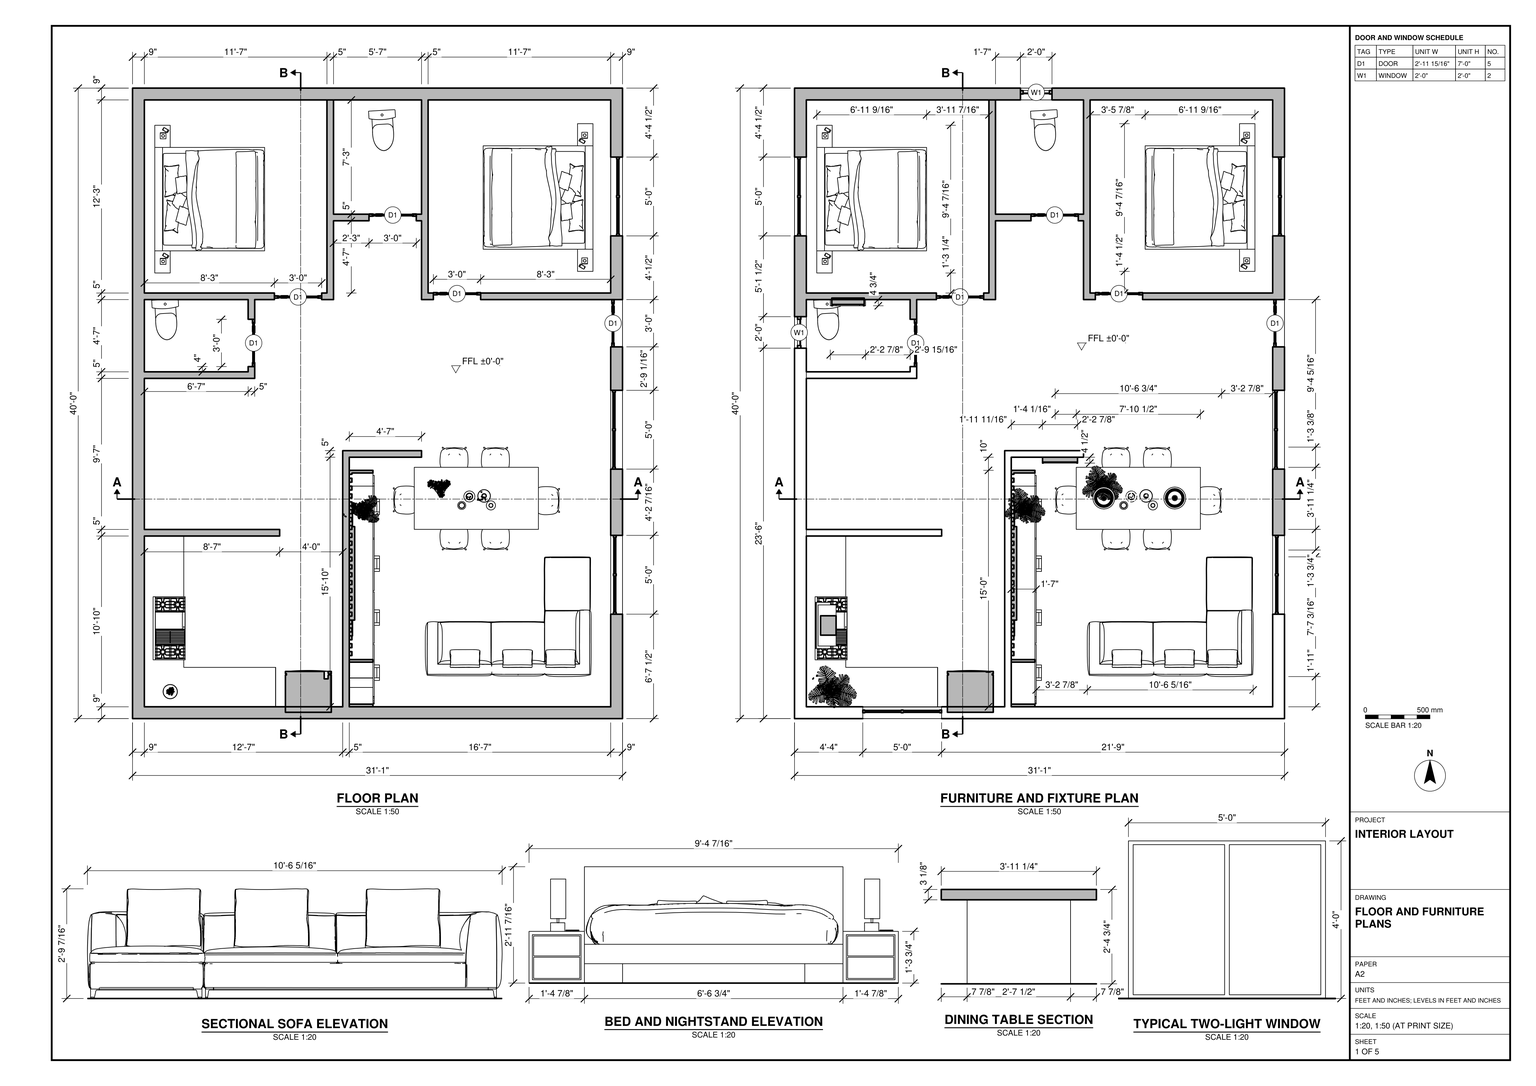
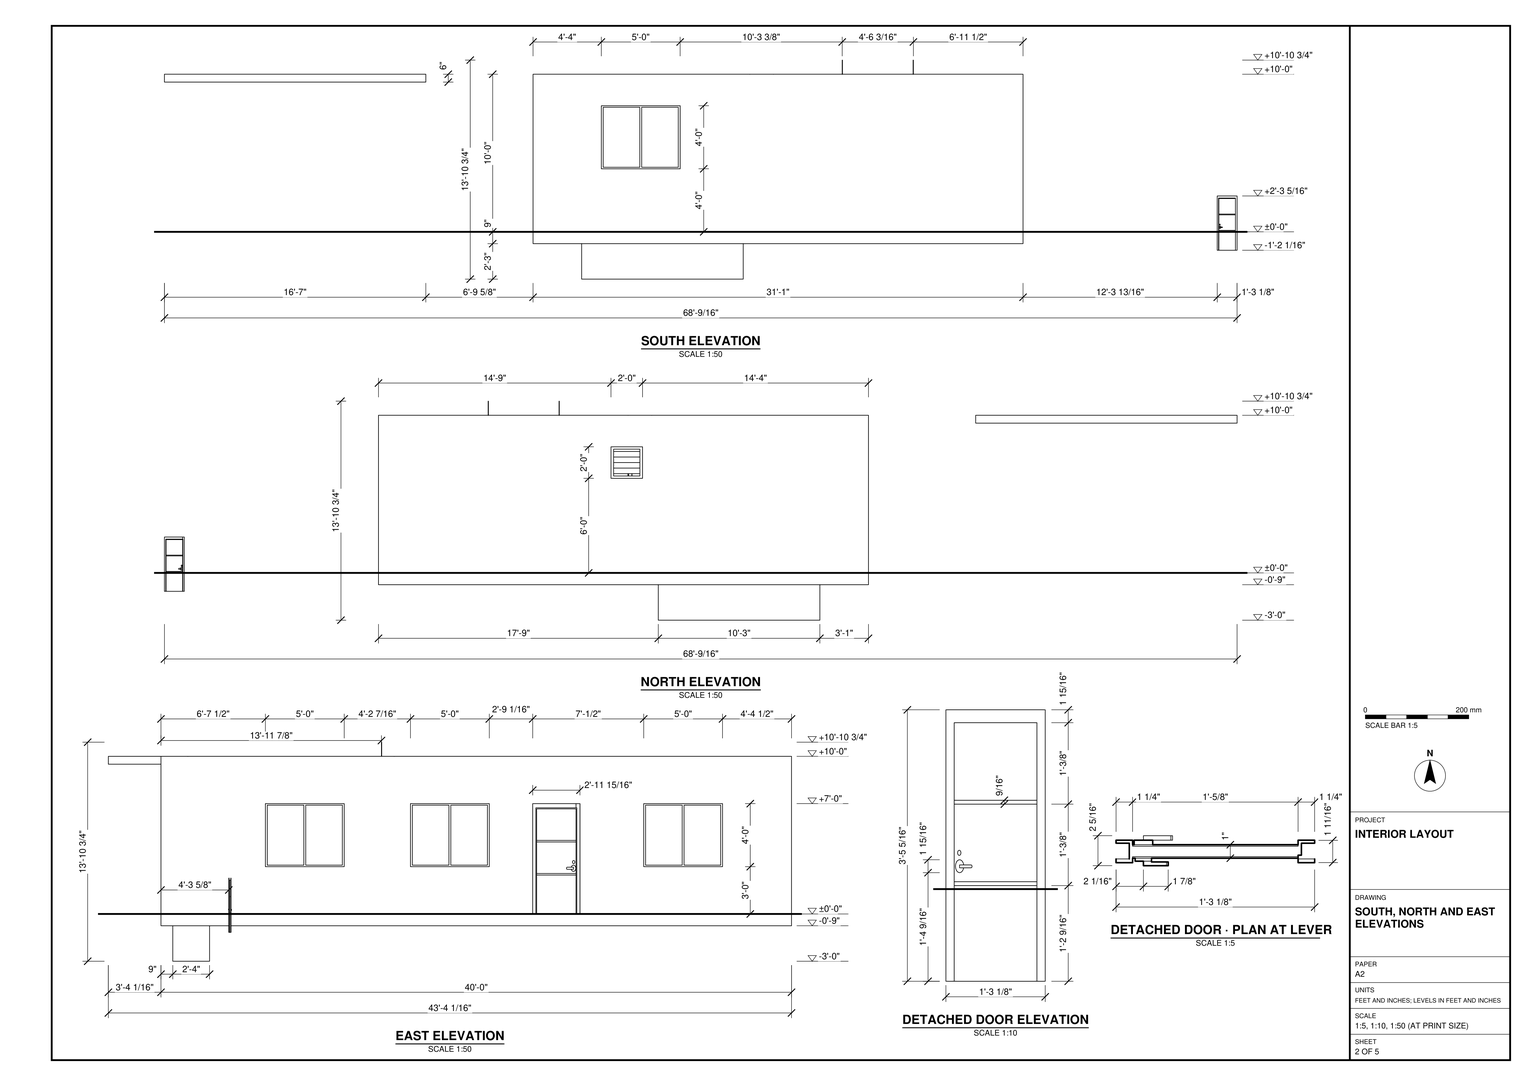
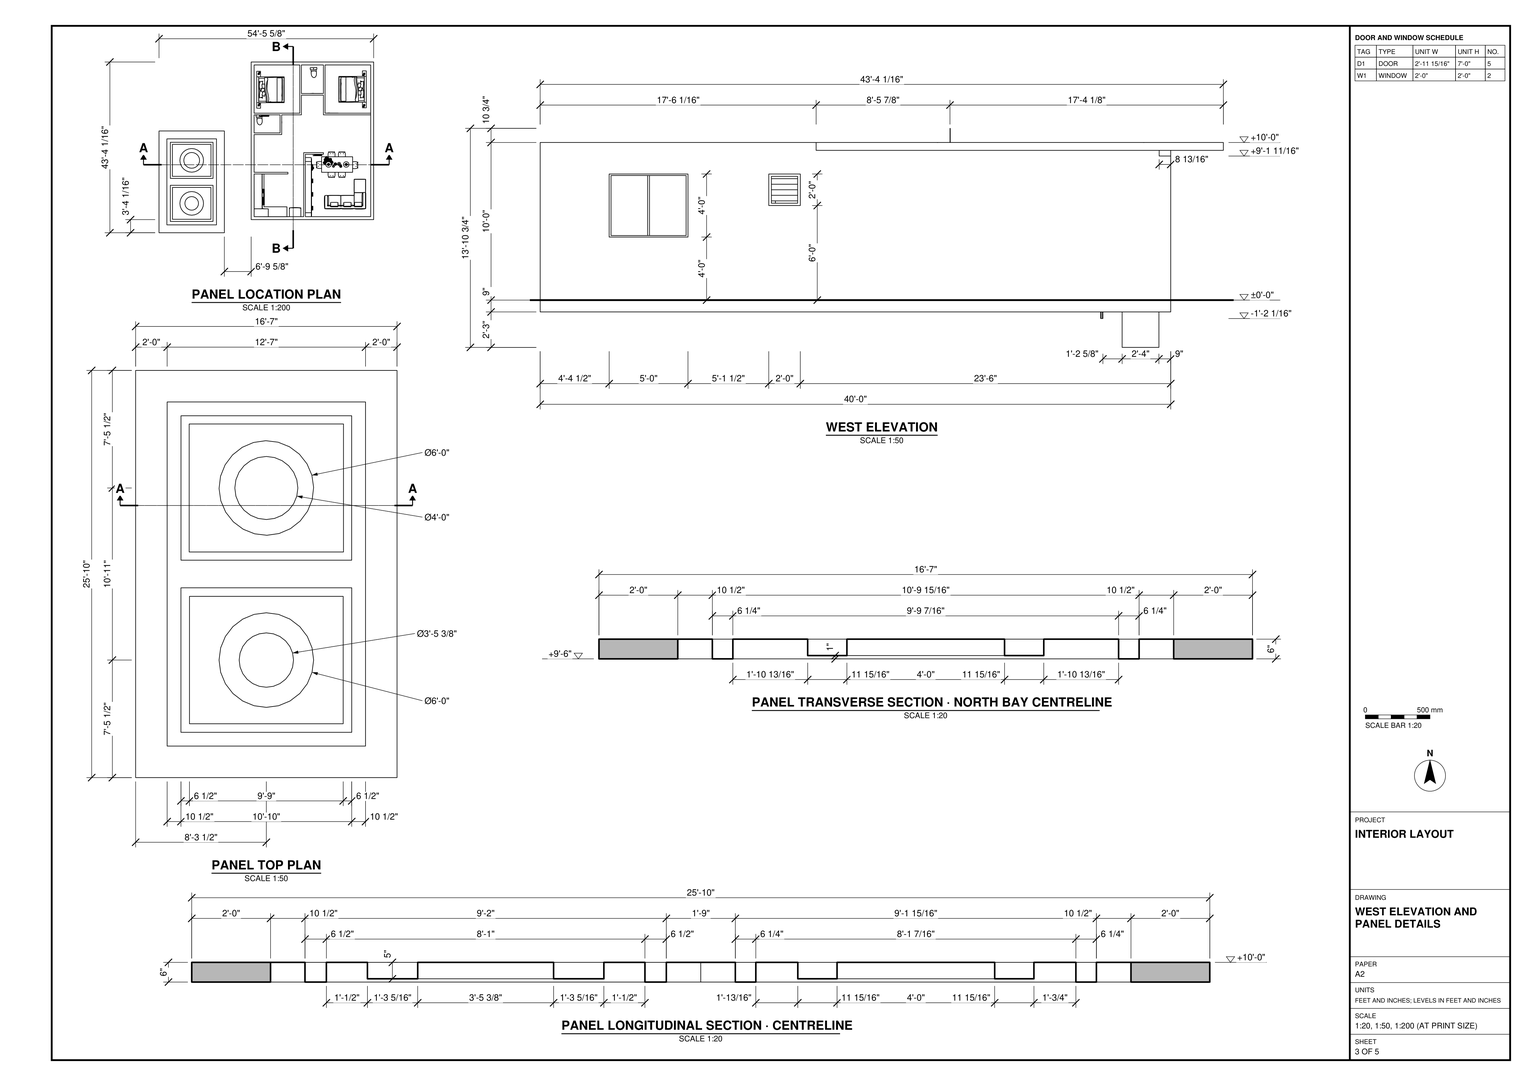
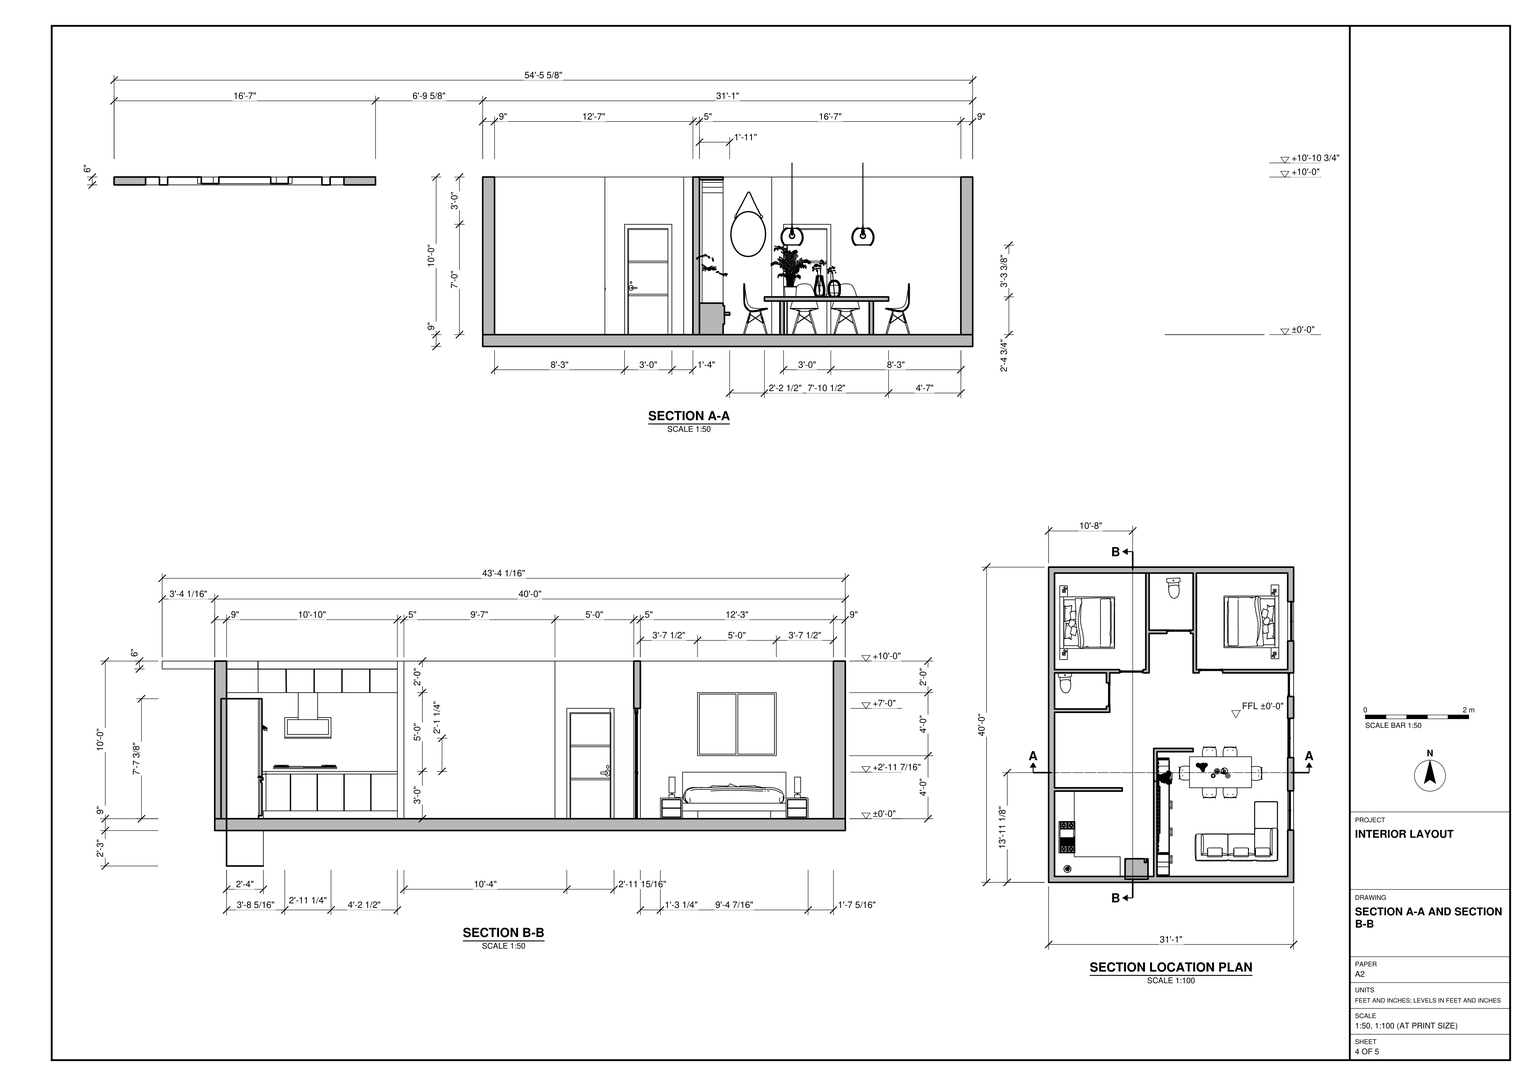
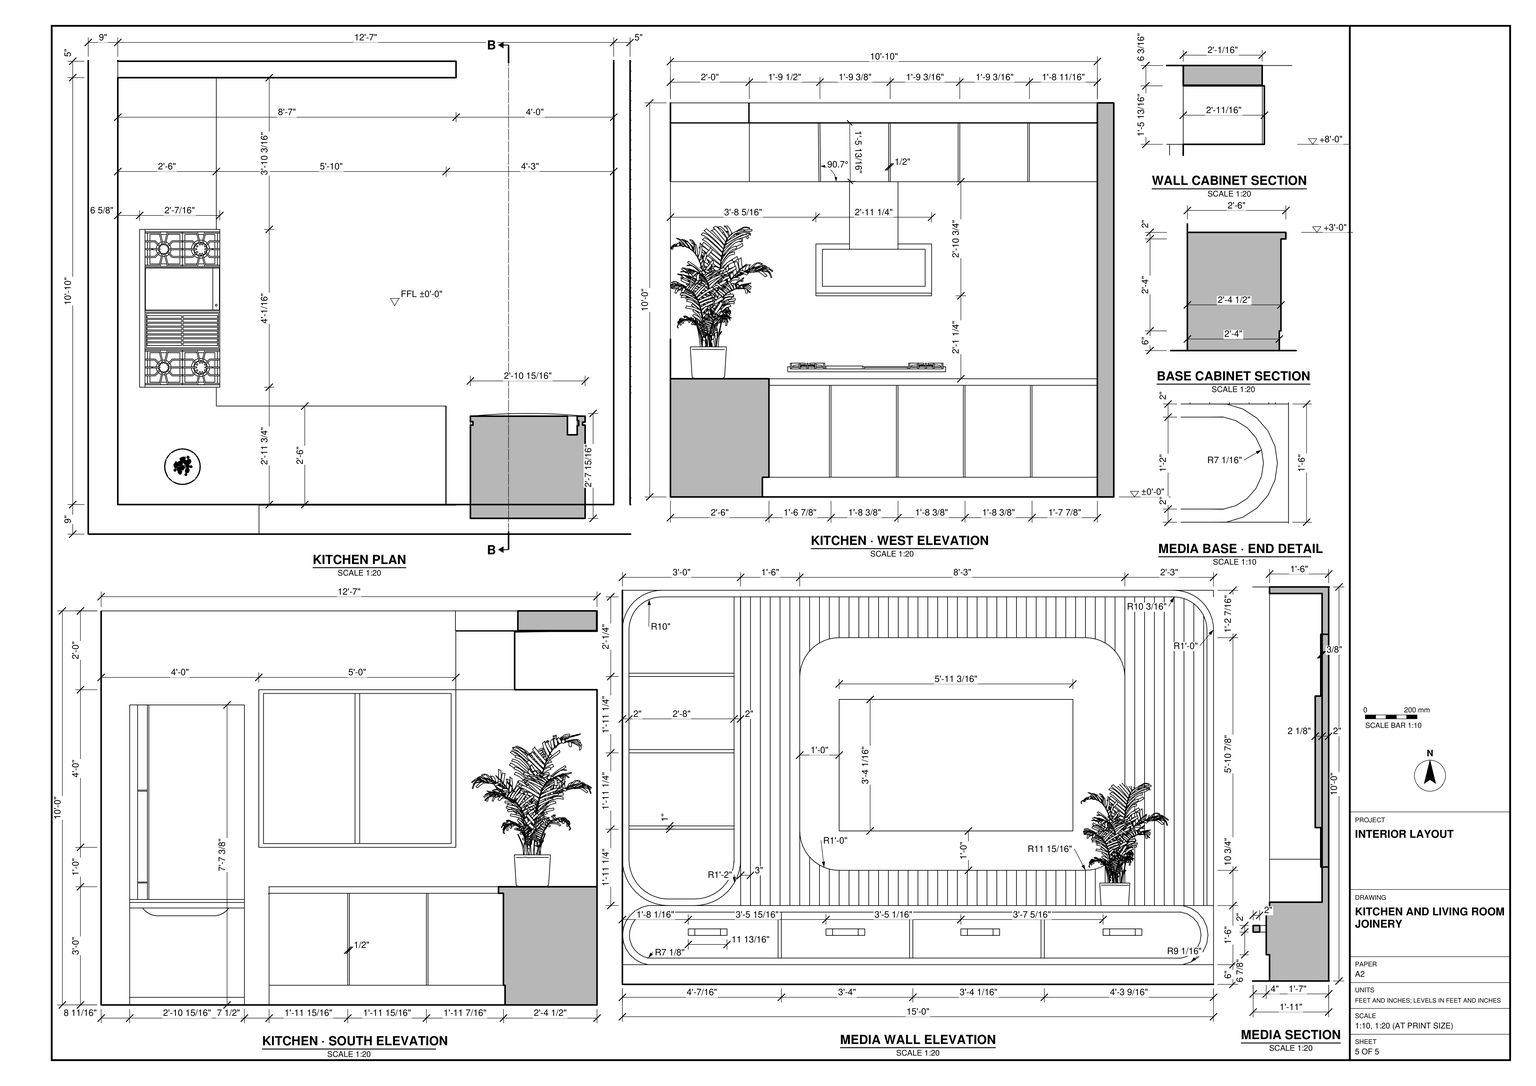
Build the interior in SketchUp from task_files/diagram_01.pdf. Work in feet and inches. Use the single finished floor level of ±0'-0". The shell measures 31'-1" east to west by 40'-0" north to south. Including the detached panel and door in their drawn positions, the overall model measures 68'-9/16" along X, 43'-4 1/16" along Y and 13'-10 3/4" along Z.

Model the floor slab, the 9" perimeter walls and the 5" partitions. Place the bedrooms in the north corners, with one toilet room between them and the other against the west wall. Follow the plans and elevations for the doors, the small high windows and the larger two-light windows. Fit out both bedrooms with beds and paired nightstands. In the southwest kitchen, arrange the counters, storage, sink and cooktop as drawn. Across the partition, place the living-area joinery, sectional sofa and dining table with chairs, keeping the passages clear as shown in plan.

Use the panel plan and sections to form the detached ceiling panel with its stepped rectangular bays and circular details. Set it west of the shell at the elevation shown, and place the separate small door east of the shell rather than fitting it into a wall. Decor and loose items, including plants, lamps, cushions and appliances, may be any suitable library components. Keep the shell elements and each furniture or joinery piece in separate groups or components, and use components for repeated parts. Save one SketchUp model as output_files/two_bedroom_interior_with_detached_ceiling_panel.skp.

# SketchUp Ruby script. Lengths in inches.
U = 1.inch
M = Sketchup.active_model
def pt(a) = Geom::Point3d.new(a.map { |v| v * U })
def face(e, loops, mat)
  f = e.add_face(loops[0].map { |a| pt(a) })
  loops[1..].each { |l| e.add_face(l.map { |a| pt(a) }).erase! }
  f.material = f.back_material = mat if mat
  f
end
# faces: each face lists its corners as indices into pts; further lists are holes
def faces(e, pts, list, mat = nil) = list.each { |f| face(e, (f[0].is_a?(Array) ? f : [f]).map { |l| l.map { |i| pts[i] } }, mat) }
# xy, xz, yz: faces in a plane at the given z, y or x. An outline is a flat list of corners, or four numbers for a rectangle; further outlines are holes
def ring(l) = l.size == 4 ? [[l[0], l[1]], [l[2], l[1]], [l[2], l[3]], [l[0], l[3]]] : l.each_slice(2).to_a
def flat(e, list, mat, &to3) = list.each { |f| face(e, (f[0].is_a?(Array) ? f : [f]).map { |l| ring(l).map { |u, v| to3.(u, v) } }, mat) }
def xy(e, z, list, mat = nil) = flat(e, list, mat) { |x, y| [x, y, z] }
def xz(e, y, list, mat = nil) = flat(e, list, mat) { |x, z| [x, y, z] }
def yz(e, x, list, mat = nil) = flat(e, list, mat) { |y, z| [x, y, z] }
def lines(e, pts, list) = list.each { |a, b| e.add_line(pt(pts[a]), pt(pts[b])) }
# prism: a flat outline (further loops are holes) pulled along v
def prism(e, loops, v, mat = nil)
  f = face(e, loops, mat); d = Geom::Vector3d.new(v.map { |x| x * U })
  f.pushpull(f.normal.samedirection?(d) ? d.length : -d.length)
end
def box(e, o, s, mat = nil) = prism(e, [[o, [o[0] + s[0], o[1], o[2]], [o[0] + s[0], o[1] + s[1], o[2]], [o[0], o[1] + s[1], o[2]]]], [0, 0, s[2]], mat)
def at(x, y, z, deg = 0) = Geom::Transformation.translation(pt([x, y, z])) * Geom::Transformation.rotation(ORIGIN, Z_AXIS, deg.degrees)
def axes(o, x, y, z) = Geom::Transformation.new([*x, 0, *y, 0, *z, 0, *pt(o).to_a, 1])
def part(name) = M.definitions.add(name)
# library, detail: a bought-in or finely detailed component or shape, given as its bounding box
def library(name, o, s) = part(name).tap { |d| box(d.entities, o, s) }
def detail(e, o, s) = box(e.add_group.entities, o, s)
def put(e, d, t, mat = nil) = e.add_instance(d, t).tap { |i| i.material = mat if mat }
def group(e, t, mat = nil) = e.add_group.tap { |g| g.transformation = t; g.material = mat if mat }.entities
root = M.entities
M.materials.add("[0008_LavenderBlush]").color = [255, 240, 245]
M.materials.add("[0022_Maroon]").color = [128, 0, 0]
M.materials.add("[0028_AntiqueWhite]").color = [250, 235, 215]
M.materials.add("[Carrera Marble]").color = [207, 207, 207]
M.materials.add("[Carrera Marble]1").color = [207, 207, 207]
M.materials.add("[Color_008]").color = [30, 30, 30]
M.materials.add("[Color_009]").color = [0, 0, 0]
M.materials.add("[Stone Marble]").color = [143, 138, 136]
M.materials.add("[Translucent Glass Gray]").color = [128, 128, 128]
M.materials["[Translucent Glass Gray]"].alpha = 0.5
M.materials.add("[Translucent Glass Tinted]1").color = [7, 201, 240]
M.materials["[Translucent Glass Tinted]1"].alpha = 0.48
M.materials.add("[Translucent_Glass_Gray]").color = [128, 128, 128]
M.materials["[Translucent_Glass_Gray]"].alpha = 0.5
M.materials.add("[Wood Cherry Original]").color = [152, 86, 42]
M.materials.add("[Wood Floor Parquet]").color = [145, 89, 39]
M.materials.add("[Wood Floor]").color = [155, 105, 61]
c1 = library("main+door",[0,-0.79,0],[47.24,7.88,82.68])
c2 = part("ventilator")
g1 = group(c2.entities,at(0,0,0))
xy(g1,0,[[0,0,24,1],[0,1,24,6.83]],"[Wood Floor Parquet]")
xy(g1,1.75,[[2,0,22,6.83]],"[Wood Floor Parquet]")
xy(g1,21.87,[[2,0,22,6.83]],"[Wood Cherry Original]")
xy(g1,23.62,[[0,0,24,1],[0,1,24,6.83]],"[Wood Floor Parquet]")
xz(g1,0,[[[0,0,24,23.62],[2,1.75,22,21.87]]],"[Wood Floor Parquet]")
xz(g1,6.83,[[[0,0,24,23.62],[2,1.75,22,21.87]]],"[Wood Cherry Original]")
yz(g1,0,[[0,0,1,23.62],[1,0,6.83,23.62]],"[Wood Floor Parquet]")
yz(g1,2,[[0,1.75,6.83,1.75,6.83,7.66,0,3.5],[0,3.5,6.83,7.66,6.83,11.8125,0,7.66],[0,7.66,6.83,11.8125,6.83,15.97,0,11.8125],[0,11.8125,6.83,15.97,6.83,20.12,0,15.97],[0,15.97,6.83,20.12,6.83,21.87,0,21.87]],"[Wood Floor Parquet]")
yz(g1,22,[[0,1.75,0,3.5,6.83,7.66,6.83,1.75],[0,3.5,0,7.66,6.83,11.8125,6.83,7.66],[0,7.66,0,11.8125,6.83,15.97,6.83,11.8125],[0,11.8125,0,15.97,6.83,20.12,6.83,15.97],[0,15.97,0,21.87,6.83,21.87,6.83,20.12]],"[Wood Floor Parquet]")
yz(g1,24,[[0,0,1,23.62],[1,0,6.83,23.62]],"[Wood Floor Parquet]")
p = [[2,0,3.5],[2,6.83,7.66],[22,6.83,7.66],[22,0,3.5],[2,6.83,11.8125],[2,0,7.66],
  [22,0,7.66],[22,6.83,11.8125],[2,0,11.8125],[2,6.83,15.97],[22,6.83,15.97],[22,0,11.8125],
  [2,6.83,20.12],[2,0,15.97],[22,0,15.97],[22,6.83,20.12]]
faces(g1,p,[[0,1,2,3],[4,5,6,7],[8,9,10,11]],"[Translucent Glass Tinted]1")
faces(g1,p,[[12,13,14,15]],"[Translucent Glass Gray]")
c3 = library("Double bed",[0,0,0],[83.59,112.46,35.43])
c4 = library("Gas cooktop",[0,0,34.52],[24.41,48.07,2.63])
c5 = part("Inclined chimney")
g2 = group(c5.entities,at(1.97,2.08,2.89))
xy(g2,0,[[0,7.9,31.3,13.68]])
xy(g2,11.29,[[0,0,31.3,13.68]])
xz(g2,13.68,[[0,0,31.3,11.29]])
yz(g2,0,[[7.9,0,0,11.29,13.68,11.29,13.68,0]])
yz(g2,31.3,[[7.9,0,13.68,0,13.68,11.29,0,11.29]])
g3 = group(c5.entities,at(0,9.85,0.4))
g4 = group(g3,at(0,0.61,0.43))
prism(g4,[[[35.24,0,0],[35.24,-3.39,4.84],[35.24,-3.58,4.7],[35.24,-0.29,0]]],[-35.24,0,0])
g5 = group(g3,at(0,-3.21,4.99))
prism(g5,[[[35.24,-0.2,-0.12],[35.24,-3.16,5],[0,-3.16,5],[0,-0.2,-0.12]]],[0,0.2,0.12])
g6 = group(g3,at(0,-6.27,10.27))
prism(g6,[[[35.24,-0.19,-0.14],[35.24,-3.58,4.7],[0,-3.58,4.7],[0,-0.19,-0.14]]],[0,0.19,0.14])
g7 = group(g3,at(0,0.61,0.43))
prism(g7,[[[35.24,0,0],[35.24,0.96,0],[35.24,-9.52,14.96],[35.24,-10.16,14.51]]],[-35.24,0,0])
g8 = group(c5.entities,at(10.24,3.95,20.8))
box(g8,[0,0,-6.62],[14.76,11.8125,20.56])
g9 = group(c5.entities,at(0,10.1,0))
prism(g9,[[[35.24,0.46,0],[35.24,1.33,0],[35.24,1.33,0.83],[35.24,1.01,0.83],[35.24,0.37,0.83],[35.24,0,0.83],[35.24,0,0.64]]],[-35.24,0,0])
c6 = part("Inclined+chimney")
put(c6.entities,c5,at(34.17,38.97,0.69))
c7 = library("Component\#33",[0,0,0],[60.64,55.48,158.625])
c8 = library("SKT_Nearly Natural 5' Kentia Palm Silk Tree",[-23.18,-17.61,0],[47.48,43.95,59.125])
c9 = library("CS300DRT",[0,0,0],[27.18,17.85,30.31])
c10 = library("Hanging wall mirror",[0,0,0],[26.88,1.18,49.49])
c11 = library("michel-club1 (1)",[-34.67,-0.85,-0.13],[126.28,91.17,33.41])
c12 = library("Modern+dining",[-0.9,-1.38,-0.1],[126.72,78.33,130.86])
c13 = library("Group\#13",[0,0,0],[23,180,120])
c14 = part("Group\#2")
xy(c14.entities,0,[[0,0,82.68,1.18]],"[Color_009]")
xy(c14.entities,1.97,[[1.97,0.98,40.35,1.18],[42.32,0.98,80.71,1.18]])
xy(c14.entities,1.97,[[1.97,0,40.35,0.3],[42.32,0,80.71,0.3]],"[Color_009]")
xy(c14.entities,80.71,[[1.97,0,40.35,0.3],[42.32,0,80.71,0.3],[1.97,0.3,40.35,0.98],[42.32,0.3,80.71,0.98],[1.97,0.98,40.35,1.18],
  [42.32,0.98,80.71,1.18]])
xy(c14.entities,82.68,[[0,0,82.68,1.18]],"[Color_008]")
xz(c14.entities,0,[[[0,0,82.68,82.68],[1.97,1.97,40.35,80.71],[42.32,1.97,80.71,80.71]]],"[Color_009]")
xz(c14.entities,0.3,[[1.97,1.97,40.35,80.71],[42.32,1.97,80.71,80.71]],"[Translucent_Glass_Gray]")
xz(c14.entities,0.98,[[1.97,1.97,40.35,80.71],[42.32,1.97,80.71,80.71]],"[Translucent_Glass_Gray]")
xz(c14.entities,1.18,[[[0,0,82.68,82.68],[1.97,1.97,80.71,80.71]],[40.35,1.97,42.32,80.71]],"[Color_009]")
yz(c14.entities,0,[[0,0,1.18,82.68]],"[Color_009]")
yz(c14.entities,1.97,[[0.98,1.97,1.18,80.71]])
yz(c14.entities,1.97,[[0,1.97,0.3,80.71]],"[Color_009]")
yz(c14.entities,40.35,[[0,1.97,0.3,80.71],[0.98,1.97,1.18,80.71]],"[Color_009]")
yz(c14.entities,42.32,[[0,1.97,0.3,80.71],[0.98,1.97,1.18,80.71]])
yz(c14.entities,80.71,[[0,1.97,0.3,80.71],[0.98,1.97,1.18,80.71]],"[Color_009]")
yz(c14.entities,82.68,[[0,0,1.18,82.68]],"[Color_009]")
xy(root,-21.97,[[317.62,49.04,440.62,77.04]])
xy(root,14.03,[[289.62,49.04,317.62,179.04],[389.48,49.04,389.62,77.04]])
xy(root,20.03,[[318.12,77.04,341.08,78.04],[341.58,77.04,365.03,78.04],[365.53,77.04,389.48,79.04],[317.62,77.54,318.12,97.44],[317.62,97.94,318.12,117.84],
  [317.62,118.34,318.12,138.24],[317.62,138.74,318.12,158.64],[317.62,159.14,318.12,179.04]])
xy(root,47.85,[[389.48,49.04,389.62,79.04]])
xy(root,48.03,[[389.48,49.04,389.62,79.04],[317.62,77.04,318.12,77.54],[341.08,77.04,341.08,78.04,318.12,78.04,318.12,79.04,365.53,79.04,365.53,77.04,365.03,77.04,365.03,78.04,341.58,78.04,341.58,77.04],[318.12,79.04,318.12,97.44,317.62,97.44,317.62,97.94,318.12,97.94,318.12,117.84,317.62,117.84,317.62,118.34,318.12,118.34,318.12,138.24,317.62,138.24,317.62,138.74,318.12,138.74,318.12,158.64,317.62,158.64,317.62,159.14,318.12,159.14,318.12,179.04,319.62,179.04,319.62,79.04]])
xy(root,50.03,[[389.48,78.6,389.51,78.6,389.48,79.04]])
xy(root,50.03,[[289.62,49.04,389.48,49.04,389.48,79.04,319.62,79.04,319.62,179.04,289.62,179.04]],"[Stone Marble]")
xy(root,128.03,[[332.62,48.84,289.62,49.04,289.74,73.04,332.74,72.84]])
xy(root,134.03,[[332.62,48.84,332.74,72.84,289.74,73.04,289.62,49.04]],"[0008_LavenderBlush]")
xz(root,49.04,[[317.62,-21.97,440.62,-21.97,440.62,14.03,389.48,14.03,389.48,47.85,389.62,47.85,389.62,48.03,389.48,48.03,389.48,50.03,317.62,50.03],[289.62,14.03,317.62,50.03]])
xz(root,77.04,[[317.62,20.03,318.12,48.03],[341.08,20.03,341.58,48.03],[365.03,20.03,365.53,48.03]])
xz(root,77.04,[[317.62,14.03,389.48,20.03]],"[Carrera Marble]1")
xz(root,77.54,[[317.62,20.03,318.12,48.03]])
xz(root,78.04,[[318.12,20.03,341.08,48.03],[341.58,20.03,365.03,48.03]],"[0028_AntiqueWhite]")
xz(root,79.04,[[365.53,20.03,365.53,48.03,389.62,48.03,389.62,47.85,389.48,47.85,389.48,20.03]],"[0028_AntiqueWhite]")
xz(root,79.04,[[319.62,48.03,389.48,50.03]],"[Stone Marble]")
xz(root,97.44,[[317.62,20.03,318.12,48.03]])
xz(root,97.94,[[317.62,20.03,318.12,48.03]])
xz(root,117.84,[[317.62,20.03,318.12,48.03]])
xz(root,118.34,[[317.62,20.03,318.12,48.03]])
xz(root,138.24,[[317.62,20.03,318.12,48.03]])
xz(root,138.74,[[317.62,20.03,318.12,48.03]])
xz(root,158.64,[[317.62,20.03,318.12,48.03]])
xz(root,159.14,[[317.62,20.03,318.12,48.03]])
xz(root,179.04,[[289.62,14.03,289.62,50.03,319.62,50.03,319.62,48.03,318.12,48.03,318.12,20.03,317.62,20.03,317.62,14.03]])
yz(root,289.62,[[49.04,14.03,179.04,50.03]])
yz(root,317.62,[[49.04,-21.97,77.04,14.03],[77.04,20.03,77.54,48.03],[97.44,20.03,97.94,48.03],[117.84,20.03,118.34,48.03],[138.24,20.03,138.74,48.03],
  [158.64,20.03,159.14,48.03]])
yz(root,317.62,[[77.04,14.03,179.04,20.03]],"[Carrera Marble]1")
yz(root,318.12,[[77.04,20.03,77.54,48.03],[77.54,20.03,78.04,48.03]])
yz(root,318.12,[[78.04,20.03,97.44,48.03],[97.94,20.03,117.84,48.03],[118.34,20.03,138.24,48.03],[138.74,20.03,158.64,48.03],[159.14,20.03,179.04,48.03]],"[0028_AntiqueWhite]")
yz(root,319.62,[[79.04,48.03,179.04,50.03]],"[Stone Marble]")
yz(root,341.08,[[77.04,20.03,78.04,48.03]])
yz(root,341.58,[[77.04,20.03,78.04,48.03]])
yz(root,365.03,[[77.04,20.03,78.04,48.03]])
yz(root,365.53,[[77.04,20.03,79.04,48.03]])
yz(root,389.48,[[49.04,14.03,77.04,14.03,77.04,20.03,79.04,20.03,79.04,47.85,49.04,47.85]],"[0028_AntiqueWhite]")
yz(root,389.48,[[49.04,48.03,79.04,50.03]],"[Stone Marble]")
yz(root,389.62,[[49.04,47.85,79.04,48.03]])
yz(root,440.62,[[49.04,-21.97,77.04,14.03]])
p = [[289.62,49.04,128.03],[332.62,48.84,128.03],[332.62,48.84,127.16],[332.62,48.84,134.03],[332.74,72.84,128.03],[332.74,72.84,134.03],
  [289.62,49.04,134.03],[289.74,73.04,134.03],[289.74,73.04,128.03],[839.5,257.66,14.03],[841.77,257.73,14.03],[848.46,258.79,14.03],
  [850.63,259.42,14.03],[852.76,260.1875,14.03],[862.45,265.92,14.03],[864.15,267.42,14.03],[836.11,377.53,14.03],[836.11,413.53,14.03],
  [839.5,291.66,14.03],[875.44,291.66,14.03],[854.83,261.09,14.03],[856.85,262.11,14.03],[858.79,263.26,14.03],[860.66,264.54,14.03],
  [846.25,258.3,14.03],[865.75,269.02,14.03],[867.24,270.71,14.03],[875.5,291.66,14.03],[875.5,293.66,14.03],[800.11,413.53,14.03],
  [800.11,377.53,14.03],[839.5,293.66,14.03],[868.63,272.5,14.03],[869.9,274.37,14.03],[871.05,276.32,14.03],[872.08,278.33,14.03],
  [872.98,280.41,14.03],[873.74,282.54,14.03],[844.02,257.94,14.03],[874.375,284.71,14.03],[874.87,286.91,14.03],[875.22,289.15,14.03],
  [875.43,291.4,14.03],[826.25,260.1875,14.03],[828.38,259.42,14.03],[830.55,258.79,14.03],[832.76,258.3,14.03],[875.5,295.66,14.03],
  [834.99,257.94,14.03],[837.24,257.73,14.03],[803.58,291.4,14.03],[803.79,289.15,14.03],[818.34,264.54,14.03],[820.21,263.26,14.03],
  [803.5,293.66,14.03],[875.22,298.17,14.03],[874.87,300.41,14.03],[839.5,295.66,14.03],[871.05,311,14.03],[869.9,312.95,14.03],
  [872.98,306.91,14.03],[872.08,308.99,14.03],[867.24,316.61,14.03],[865.75,318.3,14.03],[805.27,282.54,14.03],[806.03,280.41,14.03],
  [874.375,302.61,14.03],[873.74,304.78,14.03],[810.38,272.5,14.03],[811.77,270.71,14.03],[822.16,262.11,14.03],[864.15,319.9,14.03],
  [862.45,321.4,14.03],[860.66,322.78,14.03],[858.79,324.06,14.03],[856.85,325.21,14.03],[854.83,326.23,14.03],[850.63,327.9,14.03],
  [848.46,328.53,14.03],[841.77,329.59,14.03],[839.5,329.66,14.03],[803.57,295.66,14.03],[803.5,295.66,14.03],[809.11,274.37,14.03],
  [837.15,329.58,14.03],[834.81,329.35,14.03],[803.5,291.66,14.03],[806.93,278.33,14.03],[807.96,276.32,14.03],[868.63,314.82,14.03],
  [824.18,261.09,14.03],[852.76,327.13,14.03],[804.14,286.91,14.03],[804.64,284.71,14.03],[813.26,269.02,14.03],[814.86,267.42,14.03],
  [816.56,265.92,14.03],[875.43,295.92,14.03],[803.57,291.66,14.03],[875.44,295.66,14.03],[846.25,329.02,14.03],[844.02,329.375,14.03],
  [832.48,328.97,14.03],[830.1875,328.43,14.03],[806.24,307.4375,14.03],[805.42,305.23,14.03],[804.73,302.98,14.03],[809.57,313.66,14.03],
  [808.33,311.66,14.03],[810.94,315.58,14.03],[804.2,300.68,14.03],[817.59,322.22,14.03],[815.77,320.73,14.03],[819.5,323.59,14.03],
  [803.58,296.01,14.03],[823.58,325.95,14.03],[821.5,324.84,14.03],[812.4375,317.4,14.03],[814.05,319.12,14.03],[807.22,309.58,14.03],
  [803.8125,298.36,14.03],[827.93,327.75,14.03],[825.73,326.92,14.03],[440.62,49.04,50.03],[440.62,49.04,47.85],[389.62,77.04,50.03],
  [389.51,78.6,50.03],[440.62,78.6,50.03],[440.62,78.6,47.85],[332.62,48.84,110.03],[289.62,179.04,134.03],[289.62,179.04,128.03]]
faces(root,p,[[0,1,2],[0,6,7,8]])
faces(root,p,[[3,1,4,5],[4,8,7,5]],"[Wood Floor]")
lines(root,p,[[9,10],[11,12],[12,13],[14,15],[16,17],[18,19],[13,20],[21,22],[22,23],[24,11],[25,26],[27,28],
  [29,30],[31,18],[32,33],[33,34],[35,36],[36,37],[10,38],[17,29],[38,24],[20,21],[23,14],[15,25],
  [28,31],[34,35],[37,39],[26,32],[39,40],[30,16],[41,42],[43,44],[45,46],[47,28],[48,49],[42,19],
  [40,41],[50,51],[52,53],[54,31],[55,56],[31,57],[58,59],[60,61],[62,63],[64,65],[66,67],[68,69],
  [53,70],[63,71],[72,73],[74,75],[75,76],[77,78],[79,80],[57,81],[82,54],[83,68],[80,84],[84,85],
  [86,54],[65,87],[56,66],[87,88],[59,89],[90,43],[73,74],[76,91],[92,93],[93,64],[70,90],[44,45],
  [49,9],[69,94],[89,62],[95,96],[88,83],[97,55],[18,98],[57,99],[61,58],[71,72],[91,77],[46,48],
  [100,101],[94,95],[67,60],[101,79],[96,52],[78,100],[51,92],[28,99],[54,98],[102,103],[104,105],[105,106],
  [85,102],[107,108],[109,107],[106,110],[111,112],[113,111],[114,81],[115,116],[117,109],[118,117],[108,119],[120,114],
  [121,122],[122,115],[103,121],[116,113],[119,104],[110,120],[112,118],[19,27],[18,9],[19,28],[57,80],[81,82],
  [98,86],[99,47],[99,97],[98,50],[81,54],[123,124],[125,126],[127,128],[129,2],[6,130],[131,0]])
put(root,c1,axes([801.45,91.68,0],[0.32,0,0],[0,0.29,0],[0,0,0.5]))
put(root,c2,axes([476.62,518.14,86.03],[-1,0,0],[0,-0.38,0],[0,0,1.016]))
put(root,c3,at(547.53,380.52,14.03))
put(root,c3,at(381.16,491.75,14.03,-180))
put(root,c4,at(296.28,84.77,17.63))
put(root,c6,at(257.54,162.74,74.6,-90))
put(root,c7,axes([431.93,76.8,14.03],[-0.576,0,0],[0,-0.576,0],[0,0,0.576]))
put(root,c8,axes([309.28,60.48,50.03],[0.84,0,0],[0,0.84,0],[0,0,0.84]))
put(root,c9,axes([460.3,502.51,14.03],[0.06505,-1.12813,0],[1.12813,0.06505,0],[0,0,1.13]))
put(root,c10,axes([307.83,354.32,68.84],[1,0,0],[0,5,0],[0,0,1]))
put(root,c9,axes([295.2,358.52,14.03],[0.06505,-1.12813,0],[1.12813,0.06505,0],[0,0,1.13]))
put(root,c10,axes([469.29,234.56,73.32],[1,0,0],[0,3.79,0],[0,0,1]))
put(root,c11,at(595.09,162.35,14.17,180))
put(root,c8,axes([514.84,216.03,42.77],[0.7,0,0],[0,0.7,0],[0,0,0.7]))
put(root,c8,axes([455.94,198.88,36.79],[0.7,0,0],[0,0.7,0],[0,0,0.7]))
put(root,c12,at(479.95,169.77,14.03))
g10 = group(root,at(280.62,40.04,5.03))
xy(g10,0,[[0,0,373,480]])
xy(g10,9,[[0,0,373,480]],"[Carrera Marble]")
xz(g10,0,[[0,0,373,9]])
xz(g10,480,[[0,0,373,9]])
yz(g10,0,[[0,0,480,9]])
yz(g10,373,[[0,0,480,9]])
put(root,c13,at(445.62,49.04,14.03))
g11 = group(root,at(280.62,40.04,14.03),"[0008_LavenderBlush]")
xy(g11,0,[[0,0,0,306,9,306,9,9,51.94,9,52,8.79,52,0],[52,0,52,8.79,112,8.79,112,9,160,9,160,204,220,204,220,199,165,199,165,9,364,9,364,139.5,373,139.5,373,0],[52,8.79,51.94,9,52,9],[52,8.79,112,9],[9,139,112,144],
  [364,139.5,373,249.9375],[364,249.9375,373,283],[9,259,9,264,88,264,88,268,93,268,93,259],[88,304,93,319],[0,306,9,427.5],
  [9,319,108,324],[144,319,148,324],[148,319,153,471],[220,319,220,471,196,471,196,480,373,480,373,427.5,364,427.5,364,471,225,471,225,324,229,324,229,319],[265,319,265,324,364,324,364,427.5,373,427.5,373,319],
  [153,379,180,384],[216,379,220,384],[0,427.5,9,471],[0,471,196,480]])
xy(g11,36,[[364,79.5,373,139.5],[364,189.9375,373,249.9375],[364,367.5,373,427.5]])
xy(g11,48,[[0,367.5,9,427.5]])
xy(g11,72,[[0,282,9,306],[172,471,196,480]])
xy(g11,84,[[364,79.5,373,139.5],[364,189.9375,373,249.9375],[88,268,93,304],[364,283,373,319],[108,319,144,324],
  [229,319,265,324],[364,367.5,373,427.5],[180,379,216,384]])
xy(g11,96,[[52,0,112,8.79],[9,9,9,139,33.71,139,33.71,118.31,33.09,118.31,33.09,117.81,33.71,117.81,33.71,97.11,33.09,97.11,33.09,96.61,33.71,96.61,33.71,75.92,33.09,75.92,33.09,75.42,33.71,75.42,33.71,54.72,33.09,54.72,33.09,54.22,34.09,54.22,34.09,33.03,33.09,33.03,33.09,9],[33.09,9,52,33.03],[0,282,9,306],[0,367.5,9,427.5],
  [172,471,196,480]])
xy(g11,113.8125,[[9,9,33.09,9,33.09,33.03,34.09,33.03,34.09,54.01,33.09,54.01,33.09,54.51,33.71,54.51,33.71,75.42,33.09,75.42,33.09,75.92,33.71,75.92,33.71,96.61,33.09,96.61,33.09,97.11,33.71,97.11,33.71,117.81,33.09,117.81,33.09,118.31,33.71,118.31,33.71,139,9,139]])
xy(g11,113.8125,[[33.09,9,52,33.03]],"[Wood Floor]")
xy(g11,114,[[9.11,33,9,139,33,139.03,33.11,33.03]])
xy(g11,120,[[[0,0,373,480],[52,8.79,51.94,9,9,9,9,139,112,139,112,144,9,144,9,259,93,259,93,319,153,319,153,379,220,379,220,319,364,319,364,324,225,324,225,471,364,471,364,9,165,9,165,199,220,199,220,204,160,204,160,9,112,9,112,8.79],[9,324,148,471],[153,384,220,471],[9,264,88,319],[9.11,33,9,139,33,139.03,33,139,33.11,33.03]],[52,8.79,112,8.79,112,9,51.94,9],[9.11,33,33.11,33.03,33,139,9,139],[9,139,33,139,33,139.03]])
xz(g11,0,[[[0,0,373,120],[52,48,112,96]]])
xz(g11,9,[[9,0,9,96,52,96,52,48,112,48,112,96,52,96,52,114,9,114,9,120,160,120,160,0],[165,0,364,120],[9,113.8125,52,114]])
xz(g11,33.03,[[34.09,96,52,113.8125]],"[0028_AntiqueWhite]")
xz(g11,75.42,[[33.09,96,33.71,113.8125]])
xz(g11,75.92,[[33.09,96,33.71,113.8125]])
xz(g11,79.5,[[364,36,373,84]])
xz(g11,96.61,[[33.09,96,33.71,113.8125]])
xz(g11,97.11,[[33.09,96,33.71,113.8125]])
xz(g11,117.81,[[33.09,96,33.71,113.8125]])
xz(g11,118.31,[[33.09,96,33.71,113.8125]])
xz(g11,139,[[9,0,112,0,112,120,9,120,9,113.8125,33.71,113.8125,33.71,96,9,96],[9,96,33.71,113.8125]])
xz(g11,139.5,[[364,36,373,84]])
xz(g11,144,[[9,0,112,120]])
xz(g11,189.9375,[[364,36,373,84]])
xz(g11,199,[[165,0,220,120]])
xz(g11,204,[[160,0,220,120]])
xz(g11,249.9375,[[364,36,373,84]])
xz(g11,259,[[9,0,93,120]])
xz(g11,264,[[9,0,88,120]])
xz(g11,268,[[88,0,93,84]])
xz(g11,282,[[0,72,9,96]])
xz(g11,283,[[364,0,373,84]])
xz(g11,304,[[88,0,93,84]])
xz(g11,306,[[0,72,9,96]])
xz(g11,319,[[9,0,88,120],[93,0,108,0,108,84,144,84,144,0,153,0,153,120,93,120],[220,0,229,0,229,84,265,84,265,0,373,0,373,84,364,84,364,120,220,120]])
xz(g11,324,[[9,0,9,120,148,120,148,0,144,0,144,84,108,84,108,0],[225,0,225,120,364,120,364,0,265,0,265,84,229,84,229,0]])
xz(g11,367.5,[[364,36,373,84],[0,48,9,96]])
xz(g11,379,[[153,0,180,0,180,84,216,84,216,0,220,0,220,120,153,120]])
xz(g11,384,[[153,0,153,120,220,120,220,0,216,0,216,84,180,84,180,0]])
xz(g11,427.5,[[364,36,373,84],[0,48,9,96]])
xz(g11,471,[[9,0,148,120],[148,0,153,109.6875],[[153,0,220,120],[172,72,196,96]],[225,0,364,120]])
xz(g11,480,[[[0,0,373,120],[172,72,196,96]]])
yz(g11,0,[[[0,0,0,109.6875,8.79,109.6875,8.79,120,480,120,480,0],[367.5,48,427.5,96],[282,72,306,96]],[0,109.6875,8.79,120]])
yz(g11,9,[[9,0,139,96],[144,0,259,120],[[264,0,319,120],[282,72,306,96]],[[324,0,471,120],[367.5,48,427.5,96]],[139,96,139.9375,113.8125],
  [9,113.8125,139,120]])
yz(g11,33.09,[[54.22,96,54.72,96,54.51,113.8125,54.01,113.8125],[75.42,96,75.92,113.8125],[96.61,96,97.11,113.8125],[117.81,96,118.31,113.8125]])
yz(g11,33.71,[[54.72,96,75.42,96,75.42,113.8125,54.51,113.8125],[75.92,96,96.61,113.8125],[97.11,96,117.81,113.8125],[118.31,96,139,113.8125]],"[0028_AntiqueWhite]")
yz(g11,34.09,[[33.03,96,54.22,96,54.01,113.8125,33.03,113.8125]],"[0028_AntiqueWhite]")
yz(g11,52,[[9,96,33.03,113.8125]],"[0028_AntiqueWhite]")
yz(g11,88,[[264,0,264,120,319,120,319,0,304,0,304,84,268,84,268,0]])
yz(g11,93,[[259,0,268,0,268,84,304,84,304,0,319,0,319,120,259,120]])
yz(g11,108,[[319,0,324,84]])
yz(g11,112,[[139,0,144,120]])
yz(g11,144,[[319,0,324,84]])
yz(g11,148,[[324,0,471,120]])
yz(g11,153,[[319,0,379,120],[384,0,471,120]])
yz(g11,160,[[9,0,204,120]])
yz(g11,165,[[9,0,199,120]])
yz(g11,172,[[471,72,480,96]])
yz(g11,180,[[379,0,384,84]])
yz(g11,196,[[471,72,480,96]])
yz(g11,216,[[379,0,384,84]])
yz(g11,220,[[199,0,204,120],[319,0,379,120],[384,0,471,120]])
yz(g11,225,[[324,0,471,120]])
yz(g11,229,[[319,0,324,84]])
yz(g11,265,[[319,0,324,84]])
yz(g11,364,[[[9,0,9,120,319,120,319,84,283,84,283,0],[189.9375,36,249.9375,84],[79.5,36,139.5,84]],[[324,0,471,120],[367.5,36,427.5,84]]])
yz(g11,373,[[[0,0,283,0,283,84,319,84,319,0,480,0,480,120,0,120],[367.5,36,427.5,84],[189.9375,36,249.9375,84],[79.5,36,139.5,84]]])
p = [[33.09,54.22,96],[33.09,54.01,113.8125],[34.09,54.01,113.8125],[34.09,54.22,96],[33.09,54.51,113.8125],[33.09,54.72,96],
  [33.71,54.72,96],[33.71,54.51,113.8125],[9.11,33,120],[9,139,120],[9,139,114],[9.11,33,114],
  [33.11,33.03,114],[33.11,33.03,120],[33,139.03,120],[33,139,120],[33,139.03,114],[112,8.79,96],
  [112,9,96],[112,0,48],[112,8.79,48],[52,0,48],[52,8.79,48]]
faces(g11,p,[[0,1,2,3],[4,5,6,7],[8,9,10,11],[8,11,12,13],[10,9,14,16]])
faces(g11,p,[[14,15,13,12,16]],"[Wood Floor]")
lines(g11,p,[[17,18],[19,20],[21,22]])
put(g11,c1,axes([91.29,303.96,0],[0,-0.76125,0],[0.29,0,0],[0,0,1.016]))
put(g11,c1,axes([364.89,318.96,0],[0,-0.76125,0],[0.29,0,0],[0,0,1.016]))
put(g11,c1,axes([229.04,322.63,0],[0.76125,0,0],[0,0.29,0],[0,0,1.016]))
put(g11,c1,axes([180.15,382.47,0],[0.76125,0,0],[0,0.29,0],[0,0,1.016]))
put(g11,c1,axes([108.04,320.13,0],[0.76125,0,0],[0,0.29,0],[0,0,1.016]))
put(g11,c2,axes([2.25,306,72],[0,-1,0],[0.38,0,0],[0,0,1.016]))
put(g11,c14,axes([51.98,4.4375,48],[0.72571,0,0],[0,1.77,0],[0,0,0.58057]))
put(g11,c14,axes([367.55,189.9375,36],[0,0.72571,0],[-1.77,0,0],[0,0,0.58057]))
put(g11,c14,axes([4.5,367.5,48],[0,0.72571,0],[-1.77,0,0],[0,0,0.58057]))
put(g11,c14,axes([370.57,367.5,36],[0,0.72571,0],[-1.77,0,0],[0,0,0.58057]))
put(g11,c14,axes([368.18,79.5,36],[0,0.72571,0],[-1.77,0,0],[0,0,0.58057]))
g12 = group(root,at(0,0,134.03))
xy(g12,-6,[[[0,0,199,310],[24,24,175,286]],[[34.49,34.49,164.51,144.51],[41,41,158,138]],[[34.53,165.53,164.47,275.47],[40.77,171.77,158.23,269.23]]],"[0022_Maroon]")
xy(g12,-5,[[[99.5,53.5,90.18,54.73,81.5,58.32,74.04,64.04,68.32,71.5,64.73,80.18,63.5,89.5,64.73,98.82,68.32,107.5,74.04,114.96,81.5,120.68,90.18,124.27,99.5,125.5,108.82,124.27,117.5,120.68,124.96,114.96,130.68,107.5,134.27,98.82,135.5,89.5,134.27,80.18,130.68,71.5,124.96,64.04,117.5,58.32,108.82,54.73],[99.5,68.8125,104.85,69.52,109.84,71.58,114.13,74.87,117.42,79.16,119.48,84.15,120.1875,89.5,119.48,94.85,117.42,99.84,114.13,104.13,109.84,107.42,104.85,109.48,99.5,110.1875,94.15,109.48,89.16,107.42,84.87,104.13,81.58,99.84,79.52,94.85,78.8125,89.5,79.52,84.15,81.58,79.16,84.87,74.87,89.16,71.58,94.15,69.52]],[[99.91,184.5,90.58,185.62,81.86,189.12,74.34,194.75,68.53,202.14,64.84,210.78,63.5,220.09,64.62,229.42,68.12,238.14,73.75,245.66,81.14,251.47,89.78,255.16,99.09,256.5,108.42,255.38,117.14,251.88,124.66,246.25,130.47,238.86,134.16,230.22,135.5,220.91,134.38,211.58,130.88,202.86,125.25,195.34,117.86,189.53,109.22,185.84],[99.5,196.5,105.71,197.32,111.5,199.72,116.47,203.53,120.28,208.5,122.68,214.29,123.5,220.5,122.68,226.71,120.28,232.5,116.47,237.47,111.5,241.28,105.71,243.68,99.5,244.5,93.29,243.68,87.5,241.28,82.53,237.47,78.72,232.5,76.32,226.71,75.5,220.5,76.32,214.29,78.72,208.5,82.53,203.53,87.5,199.72,93.29,197.32]]],"[0022_Maroon]")
xy(g12,0,[[[0,0,199,310],[24,24,175,286]],[[24,24,175,286],[34.49,34.49,164.51,144.51],[34.53,165.53,164.47,275.47]],[[41,41,158,138],[99.5,53.5,108.82,54.73,117.5,58.32,124.96,64.04,130.68,71.5,134.27,80.18,135.5,89.5,134.27,98.82,130.68,107.5,124.96,114.96,117.5,120.68,108.82,124.27,99.5,125.5,90.18,124.27,81.5,120.68,74.04,114.96,68.32,107.5,64.73,98.82,63.5,89.5,64.73,80.18,68.32,71.5,74.04,64.04,81.5,58.32,90.18,54.73]],[99.5,68.8125,94.15,69.52,89.16,71.58,84.87,74.87,81.58,79.16,79.52,84.15,78.8125,89.5,79.52,94.85,81.58,99.84,84.87,104.13,89.16,107.42,94.15,109.48,99.5,110.1875,104.85,109.48,109.84,107.42,114.13,104.13,117.42,99.84,119.48,94.85,120.1875,89.5,119.48,84.15,117.42,79.16,114.13,74.87,109.84,71.58,104.85,69.52],[[40.77,171.77,158.23,269.23],[99.91,184.5,109.22,185.84,117.86,189.53,125.25,195.34,130.88,202.86,134.38,211.58,135.5,220.91,134.16,230.22,130.47,238.86,124.66,246.25,117.14,251.88,108.42,255.38,99.09,256.5,89.78,255.16,81.14,251.47,73.75,245.66,68.12,238.14,64.62,229.42,63.5,220.09,64.84,210.78,68.53,202.14,74.34,194.75,81.86,189.12,90.58,185.62]],
  [99.5,196.5,93.29,197.32,87.5,199.72,82.53,203.53,78.72,208.5,76.32,214.29,75.5,220.5,76.32,226.71,78.72,232.5,82.53,237.47,87.5,241.28,93.29,243.68,99.5,244.5,105.71,243.68,111.5,241.28,116.47,237.47,120.28,232.5,122.68,226.71,123.5,220.5,122.68,214.29,120.28,208.5,116.47,203.53,111.5,199.72,105.71,197.32]])
xz(g12,0,[[0,-6,199,0]])
xz(g12,24,[[24,-6,175,0]])
xz(g12,34.49,[[34.49,-6,164.51,0]])
xz(g12,41,[[41,-6,158,0]])
xz(g12,138,[[41,-6,158,0]])
xz(g12,144.51,[[34.49,-6,164.51,0]])
xz(g12,165.53,[[34.53,-6,164.47,0]])
xz(g12,171.77,[[40.77,-6,158.23,0]])
xz(g12,269.23,[[40.77,-6,158.23,0]])
xz(g12,275.47,[[34.53,-6,164.47,0]])
xz(g12,286,[[24,-6,175,0]])
xz(g12,310,[[0,-6,199,0]])
yz(g12,0,[[0,-6,310,0]])
yz(g12,24,[[24,-6,155,0],[155,-6,286,0]])
yz(g12,34.49,[[34.49,-6,144.51,0]])
yz(g12,34.53,[[165.53,-6,275.47,0]])
yz(g12,40.77,[[171.77,-6,269.23,0]])
yz(g12,41,[[41,-6,138,0]])
yz(g12,158,[[41,-6,138,0]])
yz(g12,158.23,[[171.77,-6,269.23,0]])
yz(g12,164.47,[[165.53,-6,275.47,0]])
yz(g12,164.51,[[34.49,-6,144.51,0]])
yz(g12,175,[[24,-6,155,0],[155,-6,286,0]])
yz(g12,199,[[0,-6,310,0]])
p = [[90.18,54.73,0],[99.5,53.5,0],[99.5,53.5,-5],[90.18,54.73,-5],[108.82,54.73,0],[108.82,54.73,-5],
  [81.5,58.32,0],[81.5,58.32,-5],[117.5,58.32,0],[117.5,58.32,-5],[74.04,64.04,0],[74.04,64.04,-5],
  [124.96,64.04,0],[124.96,64.04,-5],[68.32,71.5,0],[68.32,71.5,-5],[130.68,71.5,0],[130.68,71.5,-5],
  [99.5,68.8125,0],[94.15,69.52,0],[94.15,69.52,-5],[99.5,68.8125,-5],[104.85,69.52,0],[104.85,69.52,-5],
  [89.16,71.58,0],[89.16,71.58,-5],[109.84,71.58,0],[109.84,71.58,-5],[64.73,80.18,0],[64.73,80.18,-5],
  [134.27,80.18,0],[134.27,80.18,-5],[84.87,74.87,0],[84.87,74.87,-5],[114.13,74.87,0],[114.13,74.87,-5],
  [81.58,79.16,0],[81.58,79.16,-5],[117.42,79.16,0],[117.42,79.16,-5],[79.52,84.15,0],[79.52,84.15,-5],
  [119.48,84.15,0],[119.48,84.15,-5],[63.5,89.5,0],[63.5,89.5,-5],[135.5,89.5,0],[135.5,89.5,-5],
  [78.8125,89.5,0],[78.8125,89.5,-5],[120.1875,89.5,0],[120.1875,89.5,-5],[64.73,98.82,0],[64.73,98.82,-5],
  [79.52,94.85,0],[79.52,94.85,-5],[119.48,94.85,0],[119.48,94.85,-5],[134.27,98.82,0],[134.27,98.82,-5],
  [81.58,99.84,0],[81.58,99.84,-5],[117.42,99.84,0],[117.42,99.84,-5],[68.32,107.5,0],[68.32,107.5,-5],
  [130.68,107.5,0],[130.68,107.5,-5],[84.87,104.13,0],[84.87,104.13,-5],[114.13,104.13,0],[114.13,104.13,-5],
  [89.16,107.42,0],[89.16,107.42,-5],[109.84,107.42,0],[109.84,107.42,-5],[94.15,109.48,0],[94.15,109.48,-5],
  [104.85,109.48,0],[104.85,109.48,-5],[74.04,114.96,0],[74.04,114.96,-5],[124.96,114.96,0],[124.96,114.96,-5],
  [99.5,110.1875,0],[99.5,110.1875,-5],[81.5,120.68,0],[81.5,120.68,-5],[117.5,120.68,0],[117.5,120.68,-5],
  [90.18,124.27,0],[90.18,124.27,-5],[108.82,124.27,0],[108.82,124.27,-5],[99.5,125.5,0],[99.5,125.5,-5],
  [90.58,185.62,0],[99.91,184.5,0],[99.91,184.5,-5],[90.58,185.62,-5],[109.22,185.84,0],[109.22,185.84,-5],
  [81.86,189.12,0],[81.86,189.12,-5],[117.86,189.53,0],[117.86,189.53,-5],[74.34,194.75,0],[74.34,194.75,-5],
  [125.25,195.34,0],[125.25,195.34,-5],[68.53,202.14,0],[68.53,202.14,-5],[130.88,202.86,0],[130.88,202.86,-5],
  [99.5,196.5,0],[93.29,197.32,0],[93.29,197.32,-5],[99.5,196.5,-5],[105.71,197.32,0],[105.71,197.32,-5],
  [87.5,199.72,0],[87.5,199.72,-5],[111.5,199.72,0],[111.5,199.72,-5],[82.53,203.53,0],[82.53,203.53,-5],
  [116.47,203.53,0],[116.47,203.53,-5],[64.84,210.78,0],[64.84,210.78,-5],[134.38,211.58,0],[134.38,211.58,-5],
  [78.72,208.5,0],[78.72,208.5,-5],[120.28,208.5,0],[120.28,208.5,-5],[76.32,214.29,0],[76.32,214.29,-5],
  [122.68,214.29,0],[122.68,214.29,-5],[63.5,220.09,0],[63.5,220.09,-5],[135.5,220.91,0],[135.5,220.91,-5],
  [75.5,220.5,0],[75.5,220.5,-5],[123.5,220.5,0],[123.5,220.5,-5],[64.62,229.42,0],[64.62,229.42,-5],
  [76.32,226.71,0],[76.32,226.71,-5],[122.68,226.71,0],[122.68,226.71,-5],[134.16,230.22,0],[134.16,230.22,-5],
  [78.72,232.5,0],[78.72,232.5,-5],[120.28,232.5,0],[120.28,232.5,-5],[68.12,238.14,0],[68.12,238.14,-5],
  [130.47,238.86,0],[130.47,238.86,-5],[82.53,237.47,0],[82.53,237.47,-5],[116.47,237.47,0],[116.47,237.47,-5],
  [87.5,241.28,0],[87.5,241.28,-5],[111.5,241.28,0],[111.5,241.28,-5],[73.75,245.66,0],[73.75,245.66,-5],
  [124.66,246.25,0],[124.66,246.25,-5],[93.29,243.68,0],[93.29,243.68,-5],[105.71,243.68,0],[105.71,243.68,-5],
  [99.5,244.5,0],[99.5,244.5,-5],[81.14,251.47,0],[81.14,251.47,-5],[117.14,251.88,0],[117.14,251.88,-5],
  [89.78,255.16,0],[89.78,255.16,-5],[108.42,255.38,0],[108.42,255.38,-5],[99.09,256.5,0],[99.09,256.5,-5]]
faces(g12,p,[[0,1,2,3],[1,4,5,2],[6,0,3,7],[4,8,9,5],[10,6,7,11],[8,12,13,9],[14,10,11,15],[12,16,17,13],
  [18,19,20,21],[22,18,21,23],[19,24,25,20],[26,22,23,27],[28,14,15,29],[16,30,31,17],[24,32,33,25],[34,26,27,35],
  [32,36,37,33],[38,34,35,39],[36,40,41,37],[42,38,39,43],[44,28,29,45],[30,46,47,31],[40,48,49,41],[50,42,43,51],
  [52,44,45,53],[48,54,55,49],[56,50,51,57],[46,58,59,47],[54,60,61,55],[62,56,57,63],[64,52,53,65],[58,66,67,59],
  [60,68,69,61],[70,62,63,71],[68,72,73,69],[74,70,71,75],[72,76,77,73],[78,74,75,79],[80,64,65,81],[66,82,83,67],
  [76,84,85,77],[84,78,79,85],[86,80,81,87],[82,88,89,83],[90,86,87,91],[88,92,93,89],[94,90,91,95],[92,94,95,93],
  [96,97,98,99],[97,100,101,98],[102,96,99,103],[100,104,105,101],[106,102,103,107],[104,108,109,105],[110,106,107,111],[108,112,113,109],
  [114,115,116,117],[118,114,117,119],[115,120,121,116],[122,118,119,123],[120,124,125,121],[126,122,123,127],[128,110,111,129],[112,130,131,113],
  [124,132,133,125],[134,126,127,135],[132,136,137,133],[138,134,135,139],[140,128,129,141],[130,142,143,131],[136,144,145,137],[146,138,139,147],
  [148,140,141,149],[144,150,151,145],[152,146,147,153],[142,154,155,143],[150,156,157,151],[158,152,153,159],[160,148,149,161],[154,162,163,155],
  [156,164,165,157],[166,158,159,167],[164,168,169,165],[170,166,167,171],[172,160,161,173],[162,174,175,163],[168,176,177,169],[178,170,171,179],
  [176,180,181,177],[180,178,179,181],[182,172,173,183],[174,184,185,175],[186,182,183,187],[184,188,189,185],[190,186,187,191],[188,190,191,189]])
